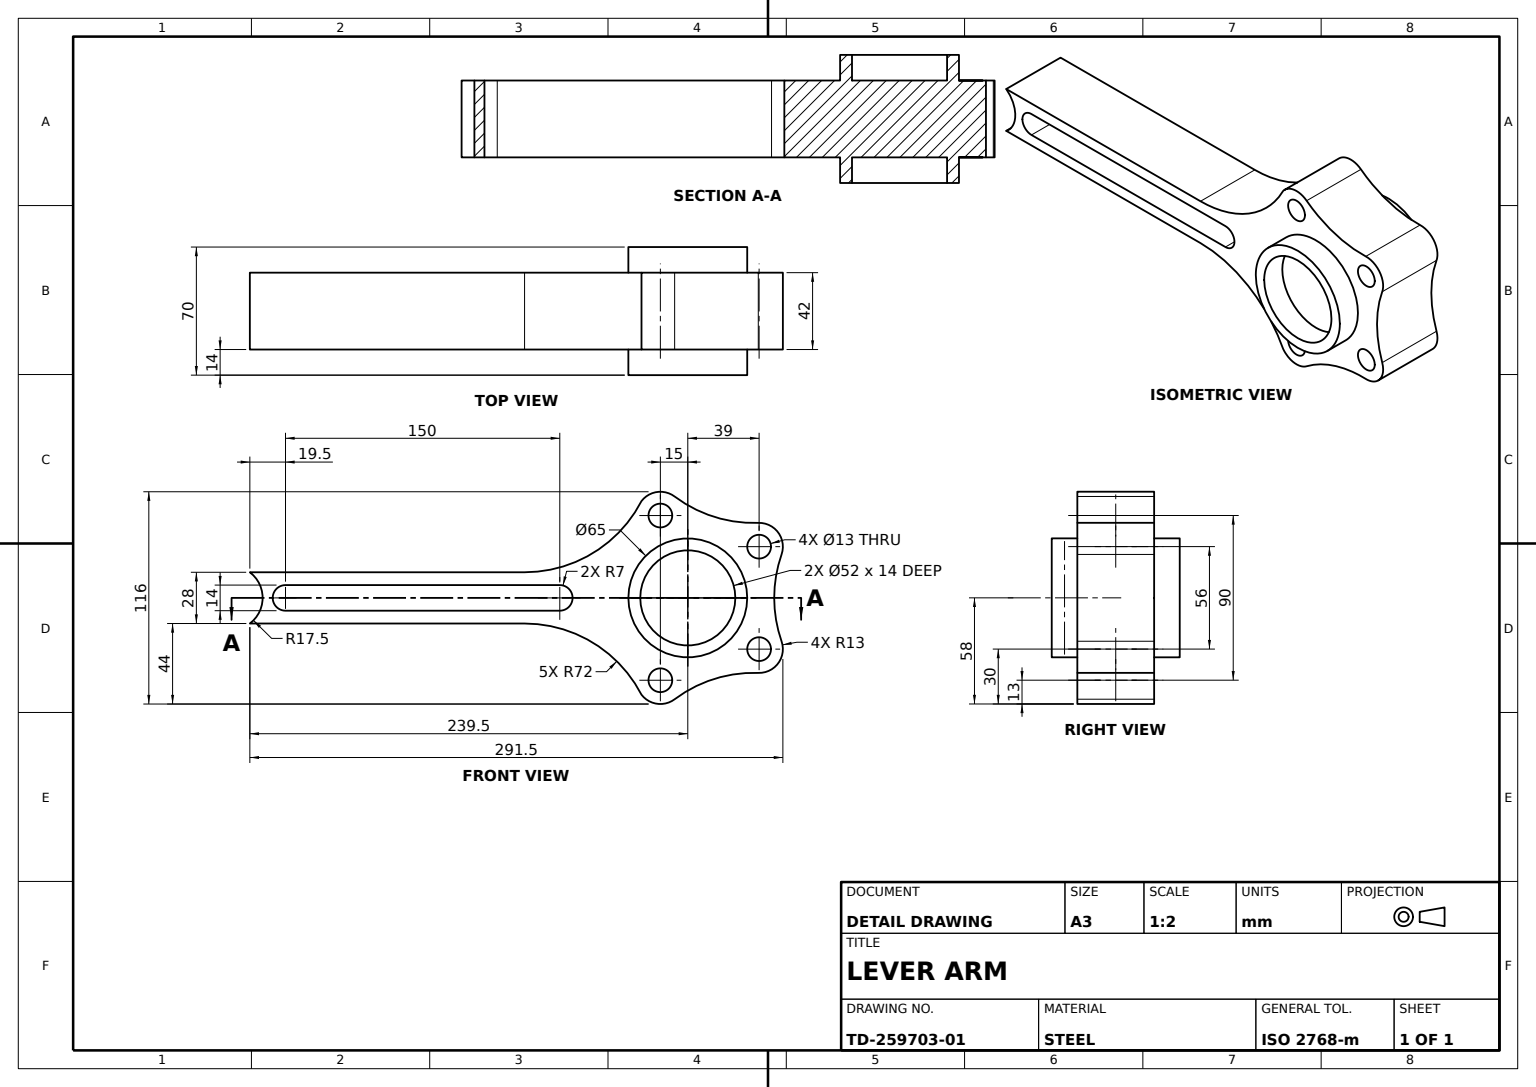
ISO-10303-21;
HEADER;
FILE_DESCRIPTION((''),'2;1');
FILE_NAME('','',(''),(''),'','','');
FILE_SCHEMA(('AUTOMOTIVE_DESIGN'));
ENDSEC;
DATA;
#1=APPLICATION_CONTEXT('');
#2=PRODUCT_CONTEXT('',#1,'mechanical');
#3=PRODUCT('','','',(#2));
#4=PRODUCT_DEFINITION_FORMATION('','',#3);
#5=PRODUCT_DEFINITION_CONTEXT('',#1,'design');
#6=PRODUCT_DEFINITION('','',#4,#5);
#7=PRODUCT_DEFINITION_SHAPE('','',#6);
#8=(LENGTH_UNIT()NAMED_UNIT(*)SI_UNIT(.MILLI.,.METRE.));
#9=(NAMED_UNIT(*)PLANE_ANGLE_UNIT()SI_UNIT($,.RADIAN.));
#10=(NAMED_UNIT(*)SI_UNIT($,.STERADIAN.)SOLID_ANGLE_UNIT());
#11=UNCERTAINTY_MEASURE_WITH_UNIT(LENGTH_MEASURE(1.E-05),#8,'distance_accuracy_value','');
#12=(GEOMETRIC_REPRESENTATION_CONTEXT(3)GLOBAL_UNCERTAINTY_ASSIGNED_CONTEXT((#11))GLOBAL_UNIT_ASSIGNED_CONTEXT((#8,#9,#10))REPRESENTATION_CONTEXT('',''));
#13=CARTESIAN_POINT('',(-70.,-7.,21.));
#14=VERTEX_POINT('',#13);
#15=CARTESIAN_POINT('',(-220.,-7.,21.));
#16=VERTEX_POINT('',#15);
#17=CARTESIAN_POINT('',(0.,-7.,21.));
#18=DIRECTION('',(-1.,0.,0.));
#19=VECTOR('',#18,1000.);
#20=LINE('',#17,#19);
#21=EDGE_CURVE('',#14,#16,#20,.T.);
#22=ORIENTED_EDGE('',*,*,#21,.F.);
#23=CARTESIAN_POINT('',(-70.,-7.,-21.));
#24=VERTEX_POINT('',#23);
#25=DIRECTION('',(0.,0.,-1.));
#26=VECTOR('',#25,1000.);
#27=LINE('',#13,#26);
#28=EDGE_CURVE('',#14,#24,#27,.T.);
#29=ORIENTED_EDGE('',*,*,#28,.T.);
#30=CARTESIAN_POINT('',(-220.,-7.,-21.));
#31=VERTEX_POINT('',#30);
#32=CARTESIAN_POINT('',(0.,-7.,-21.));
#33=LINE('',#32,#19);
#34=EDGE_CURVE('',#24,#31,#33,.T.);
#35=ORIENTED_EDGE('',*,*,#34,.T.);
#36=LINE('',#15,#26);
#37=EDGE_CURVE('',#16,#31,#36,.T.);
#38=ORIENTED_EDGE('',*,*,#37,.F.);
#39=EDGE_LOOP('',(#22,#29,#35,#38));
#40=FACE_OUTER_BOUND('',#39,.T.);
#41=DIRECTION('',(0.,-1.,0.));
#42=AXIS2_PLACEMENT_3D('',#17,#41,#25);
#43=PLANE('',#42);
#44=ADVANCED_FACE('',(#40),#43,.F.);
#45=CARTESIAN_POINT('',(26.,0.,-21.));
#46=VERTEX_POINT('',#45);
#47=CARTESIAN_POINT('',(26.,0.,-35.));
#48=VERTEX_POINT('',#47);
#49=CARTESIAN_POINT('',(26.,0.,35.));
#50=LINE('',#49,#26);
#51=EDGE_CURVE('',#46,#48,#50,.T.);
#52=ORIENTED_EDGE('',*,*,#51,.F.);
#53=CARTESIAN_POINT('',(-26.,0.,-21.));
#54=VERTEX_POINT('',#53);
#55=CARTESIAN_POINT('',(0.,0.,-21.));
#56=AXIS2_PLACEMENT_3D('',#55,#25,#18);
#57=CIRCLE('',#56,26.);
#58=EDGE_CURVE('',#54,#46,#57,.T.);
#59=ORIENTED_EDGE('',*,*,#58,.F.);
#60=CARTESIAN_POINT('',(-26.,0.,-35.));
#61=VERTEX_POINT('',#60);
#62=CARTESIAN_POINT('',(-26.,0.,35.));
#63=LINE('',#62,#26);
#64=EDGE_CURVE('',#54,#61,#63,.T.);
#65=ORIENTED_EDGE('',*,*,#64,.T.);
#66=CARTESIAN_POINT('',(0.,0.,-35.));
#67=DIRECTION('',(0.,0.,1.));
#68=DIRECTION('',(1.,0.,0.));
#69=AXIS2_PLACEMENT_3D('',#66,#67,#68);
#70=CIRCLE('',#69,26.);
#71=EDGE_CURVE('',#48,#61,#70,.T.);
#72=ORIENTED_EDGE('',*,*,#71,.F.);
#73=EDGE_LOOP('',(#52,#59,#65,#72));
#74=FACE_OUTER_BOUND('',#73,.T.);
#75=CARTESIAN_POINT('',(0.,0.,35.));
#76=AXIS2_PLACEMENT_3D('',#75,#25,#18);
#77=CYLINDRICAL_SURFACE('',#76,26.);
#78=ADVANCED_FACE('',(#74),#77,.F.);
#79=ORIENTED_EDGE('',*,*,#71,.T.);
#80=EDGE_CURVE('',#61,#48,#70,.T.);
#81=ORIENTED_EDGE('',*,*,#80,.T.);
#82=EDGE_LOOP('',(#79,#81));
#83=FACE_BOUND('',#82,.T.);
#84=CARTESIAN_POINT('',(-32.5,0.,-35.));
#85=VERTEX_POINT('',#84);
#86=CARTESIAN_POINT('',(32.5,0.,-35.));
#87=VERTEX_POINT('',#86);
#88=CIRCLE('',#69,32.5);
#89=EDGE_CURVE('',#85,#87,#88,.T.);
#90=ORIENTED_EDGE('',*,*,#89,.F.);
#91=EDGE_CURVE('',#87,#85,#88,.T.);
#92=ORIENTED_EDGE('',*,*,#91,.F.);
#93=EDGE_LOOP('',(#90,#92));
#94=FACE_OUTER_BOUND('',#93,.T.);
#95=PLANE('',#69);
#96=ADVANCED_FACE('',(#83,#94),#95,.F.);
#97=CARTESIAN_POINT('',(-89.262059,-14.,21.));
#98=VERTEX_POINT('',#97);
#99=CARTESIAN_POINT('',(-25.315909,-52.91088,21.));
#100=VERTEX_POINT('',#99);
#101=CARTESIAN_POINT('',(-89.262059,-86.,21.));
#102=AXIS2_PLACEMENT_3D('',#101,#25,#18);
#103=CIRCLE('',#102,72.);
#104=EDGE_CURVE('',#98,#100,#103,.T.);
#105=ORIENTED_EDGE('',*,*,#104,.F.);
#106=CARTESIAN_POINT('',(-89.262059,-14.,-21.));
#107=VERTEX_POINT('',#106);
#108=LINE('',#97,#26);
#109=EDGE_CURVE('',#98,#107,#108,.T.);
#110=ORIENTED_EDGE('',*,*,#109,.T.);
#111=CARTESIAN_POINT('',(-25.315909,-52.91088,-21.));
#112=VERTEX_POINT('',#111);
#113=CARTESIAN_POINT('',(-89.262059,-86.,-21.));
#114=AXIS2_PLACEMENT_3D('',#113,#25,#18);
#115=CIRCLE('',#114,72.);
#116=EDGE_CURVE('',#107,#112,#115,.T.);
#117=ORIENTED_EDGE('',*,*,#116,.T.);
#118=LINE('',#99,#26);
#119=EDGE_CURVE('',#100,#112,#118,.T.);
#120=ORIENTED_EDGE('',*,*,#119,.F.);
#121=EDGE_LOOP('',(#105,#110,#117,#120));
#122=FACE_OUTER_BOUND('',#121,.T.);
#123=CYLINDRICAL_SURFACE('',#102,72.);
#124=ADVANCED_FACE('',(#122),#123,.F.);
#125=CARTESIAN_POINT('',(45.5,-28.,21.));
#126=VERTEX_POINT('',#125);
#127=CARTESIAN_POINT('',(45.5,-28.,-21.));
#128=VERTEX_POINT('',#127);
#129=LINE('',#125,#26);
#130=EDGE_CURVE('',#126,#128,#129,.T.);
#131=ORIENTED_EDGE('',*,*,#130,.T.);
#132=CARTESIAN_POINT('',(32.5,-28.,-21.));
#133=VERTEX_POINT('',#132);
#134=CARTESIAN_POINT('',(39.,-28.,-21.));
#135=AXIS2_PLACEMENT_3D('',#134,#25,#18);
#136=CIRCLE('',#135,6.5);
#137=EDGE_CURVE('',#128,#133,#136,.T.);
#138=ORIENTED_EDGE('',*,*,#137,.T.);
#139=CARTESIAN_POINT('',(32.5,-28.,21.));
#140=VERTEX_POINT('',#139);
#141=LINE('',#139,#26);
#142=EDGE_CURVE('',#140,#133,#141,.T.);
#143=ORIENTED_EDGE('',*,*,#142,.F.);
#144=CARTESIAN_POINT('',(39.,-28.,21.));
#145=AXIS2_PLACEMENT_3D('',#144,#25,#18);
#146=CIRCLE('',#145,6.5);
#147=EDGE_CURVE('',#126,#140,#146,.T.);
#148=ORIENTED_EDGE('',*,*,#147,.F.);
#149=EDGE_LOOP('',(#131,#138,#143,#148));
#150=FACE_OUTER_BOUND('',#149,.T.);
#151=CYLINDRICAL_SURFACE('',#145,6.5);
#152=ADVANCED_FACE('',(#150),#151,.F.);
#153=CARTESIAN_POINT('',(-7.189691,-55.392261,21.));
#154=VERTEX_POINT('',#153);
#155=CARTESIAN_POINT('',(-7.189691,-55.392261,-21.));
#156=VERTEX_POINT('',#155);
#157=LINE('',#153,#26);
#158=EDGE_CURVE('',#154,#156,#157,.T.);
#159=ORIENTED_EDGE('',*,*,#158,.T.);
#160=CARTESIAN_POINT('',(38.551485,-40.992261,-21.));
#161=VERTEX_POINT('',#160);
#162=CARTESIAN_POINT('',(36.067402,-112.949396,-21.));
#163=AXIS2_PLACEMENT_3D('',#162,#25,#18);
#164=CIRCLE('',#163,72.);
#165=EDGE_CURVE('',#156,#161,#164,.T.);
#166=ORIENTED_EDGE('',*,*,#165,.T.);
#167=CARTESIAN_POINT('',(38.551485,-40.992261,21.));
#168=VERTEX_POINT('',#167);
#169=LINE('',#167,#26);
#170=EDGE_CURVE('',#168,#161,#169,.T.);
#171=ORIENTED_EDGE('',*,*,#170,.F.);
#172=CARTESIAN_POINT('',(36.067402,-112.949396,21.));
#173=AXIS2_PLACEMENT_3D('',#172,#25,#18);
#174=CIRCLE('',#173,72.);
#175=EDGE_CURVE('',#154,#168,#174,.T.);
#176=ORIENTED_EDGE('',*,*,#175,.F.);
#177=EDGE_LOOP('',(#159,#166,#171,#176));
#178=FACE_OUTER_BOUND('',#177,.T.);
#179=CYLINDRICAL_SURFACE('',#173,72.);
#180=ADVANCED_FACE('',(#178),#179,.F.);
#181=EDGE_CURVE('',#46,#54,#57,.T.);
#182=ORIENTED_EDGE('',*,*,#181,.T.);
#183=ORIENTED_EDGE('',*,*,#58,.T.);
#184=EDGE_LOOP('',(#182,#183));
#185=FACE_OUTER_BOUND('',#184,.T.);
#186=PLANE('',#56);
#187=ADVANCED_FACE('',(#185),#186,.T.);
#188=CARTESIAN_POINT('',(-25.315909,52.91088,21.));
#189=VERTEX_POINT('',#188);
#190=CARTESIAN_POINT('',(-7.189691,55.392261,21.));
#191=VERTEX_POINT('',#190);
#192=CARTESIAN_POINT('',(-15.,45.,21.));
#193=AXIS2_PLACEMENT_3D('',#192,#25,#18);
#194=CIRCLE('',#193,13.);
#195=EDGE_CURVE('',#189,#191,#194,.T.);
#196=ORIENTED_EDGE('',*,*,#195,.T.);
#197=CARTESIAN_POINT('',(-7.189691,55.392261,-21.));
#198=VERTEX_POINT('',#197);
#199=LINE('',#190,#26);
#200=EDGE_CURVE('',#191,#198,#199,.T.);
#201=ORIENTED_EDGE('',*,*,#200,.T.);
#202=CARTESIAN_POINT('',(-25.315909,52.91088,-21.));
#203=VERTEX_POINT('',#202);
#204=CARTESIAN_POINT('',(-15.,45.,-21.));
#205=AXIS2_PLACEMENT_3D('',#204,#25,#18);
#206=CIRCLE('',#205,13.);
#207=EDGE_CURVE('',#203,#198,#206,.T.);
#208=ORIENTED_EDGE('',*,*,#207,.F.);
#209=LINE('',#188,#26);
#210=EDGE_CURVE('',#189,#203,#209,.T.);
#211=ORIENTED_EDGE('',*,*,#210,.F.);
#212=EDGE_LOOP('',(#196,#201,#208,#211));
#213=FACE_OUTER_BOUND('',#212,.T.);
#214=CYLINDRICAL_SURFACE('',#193,13.);
#215=ADVANCED_FACE('',(#213),#214,.T.);
#216=CARTESIAN_POINT('',(-21.5,-45.,-21.));
#217=VERTEX_POINT('',#216);
#218=CARTESIAN_POINT('',(-8.5,-45.,-21.));
#219=VERTEX_POINT('',#218);
#220=CARTESIAN_POINT('',(-15.,-45.,-21.));
#221=AXIS2_PLACEMENT_3D('',#220,#25,#18);
#222=CIRCLE('',#221,6.5);
#223=EDGE_CURVE('',#217,#219,#222,.T.);
#224=ORIENTED_EDGE('',*,*,#223,.T.);
#225=CARTESIAN_POINT('',(-8.5,-45.,21.));
#226=VERTEX_POINT('',#225);
#227=LINE('',#225,#26);
#228=EDGE_CURVE('',#226,#219,#227,.T.);
#229=ORIENTED_EDGE('',*,*,#228,.F.);
#230=CARTESIAN_POINT('',(-21.5,-45.,21.));
#231=VERTEX_POINT('',#230);
#232=CARTESIAN_POINT('',(-15.,-45.,21.));
#233=AXIS2_PLACEMENT_3D('',#232,#25,#18);
#234=CIRCLE('',#233,6.5);
#235=EDGE_CURVE('',#231,#226,#234,.T.);
#236=ORIENTED_EDGE('',*,*,#235,.F.);
#237=LINE('',#230,#26);
#238=EDGE_CURVE('',#231,#217,#237,.T.);
#239=ORIENTED_EDGE('',*,*,#238,.T.);
#240=EDGE_LOOP('',(#224,#229,#236,#239));
#241=FACE_OUTER_BOUND('',#240,.T.);
#242=CYLINDRICAL_SURFACE('',#233,6.5);
#243=ADVANCED_FACE('',(#241),#242,.F.);
#244=CARTESIAN_POINT('',(32.5,28.,21.));
#245=VERTEX_POINT('',#244);
#246=CARTESIAN_POINT('',(45.5,28.,21.));
#247=VERTEX_POINT('',#246);
#248=CARTESIAN_POINT('',(39.,28.,21.));
#249=AXIS2_PLACEMENT_3D('',#248,#25,#18);
#250=CIRCLE('',#249,6.5);
#251=EDGE_CURVE('',#245,#247,#250,.T.);
#252=ORIENTED_EDGE('',*,*,#251,.F.);
#253=CARTESIAN_POINT('',(32.5,28.,-21.));
#254=VERTEX_POINT('',#253);
#255=LINE('',#244,#26);
#256=EDGE_CURVE('',#245,#254,#255,.T.);
#257=ORIENTED_EDGE('',*,*,#256,.T.);
#258=CARTESIAN_POINT('',(45.5,28.,-21.));
#259=VERTEX_POINT('',#258);
#260=CARTESIAN_POINT('',(39.,28.,-21.));
#261=AXIS2_PLACEMENT_3D('',#260,#25,#18);
#262=CIRCLE('',#261,6.5);
#263=EDGE_CURVE('',#254,#259,#262,.T.);
#264=ORIENTED_EDGE('',*,*,#263,.T.);
#265=LINE('',#246,#26);
#266=EDGE_CURVE('',#247,#259,#265,.T.);
#267=ORIENTED_EDGE('',*,*,#266,.F.);
#268=EDGE_LOOP('',(#252,#257,#264,#267));
#269=FACE_OUTER_BOUND('',#268,.T.);
#270=CYLINDRICAL_SURFACE('',#249,6.5);
#271=ADVANCED_FACE('',(#269),#270,.F.);
#272=ORIENTED_EDGE('',*,*,#238,.F.);
#273=EDGE_CURVE('',#226,#231,#234,.T.);
#274=ORIENTED_EDGE('',*,*,#273,.F.);
#275=ORIENTED_EDGE('',*,*,#228,.T.);
#276=EDGE_CURVE('',#219,#217,#222,.T.);
#277=ORIENTED_EDGE('',*,*,#276,.T.);
#278=EDGE_LOOP('',(#272,#274,#275,#277));
#279=FACE_OUTER_BOUND('',#278,.T.);
#280=ADVANCED_FACE('',(#279),#242,.F.);
#281=ORIENTED_EDGE('',*,*,#37,.T.);
#282=CARTESIAN_POINT('',(-227.,0.,-21.));
#283=VERTEX_POINT('',#282);
#284=CARTESIAN_POINT('',(-220.,0.,-21.));
#285=AXIS2_PLACEMENT_3D('',#284,#25,#18);
#286=CIRCLE('',#285,7.);
#287=EDGE_CURVE('',#31,#283,#286,.T.);
#288=ORIENTED_EDGE('',*,*,#287,.T.);
#289=CARTESIAN_POINT('',(-227.,0.,21.));
#290=VERTEX_POINT('',#289);
#291=LINE('',#289,#26);
#292=EDGE_CURVE('',#290,#283,#291,.T.);
#293=ORIENTED_EDGE('',*,*,#292,.F.);
#294=CARTESIAN_POINT('',(-220.,0.,21.));
#295=AXIS2_PLACEMENT_3D('',#294,#25,#18);
#296=CIRCLE('',#295,7.);
#297=EDGE_CURVE('',#16,#290,#296,.T.);
#298=ORIENTED_EDGE('',*,*,#297,.F.);
#299=EDGE_LOOP('',(#281,#288,#293,#298));
#300=FACE_OUTER_BOUND('',#299,.T.);
#301=CYLINDRICAL_SURFACE('',#295,7.);
#302=ADVANCED_FACE('',(#300),#301,.F.);
#303=CARTESIAN_POINT('',(-89.262059,14.,-21.));
#304=VERTEX_POINT('',#303);
#305=CARTESIAN_POINT('',(-89.262059,86.,-21.));
#306=AXIS2_PLACEMENT_3D('',#305,#25,#18);
#307=CIRCLE('',#306,72.);
#308=EDGE_CURVE('',#203,#304,#307,.T.);
#309=ORIENTED_EDGE('',*,*,#308,.T.);
#310=CARTESIAN_POINT('',(-89.262059,14.,21.));
#311=VERTEX_POINT('',#310);
#312=LINE('',#310,#26);
#313=EDGE_CURVE('',#311,#304,#312,.T.);
#314=ORIENTED_EDGE('',*,*,#313,.F.);
#315=CARTESIAN_POINT('',(-89.262059,86.,21.));
#316=AXIS2_PLACEMENT_3D('',#315,#25,#18);
#317=CIRCLE('',#316,72.);
#318=EDGE_CURVE('',#189,#311,#317,.T.);
#319=ORIENTED_EDGE('',*,*,#318,.F.);
#320=ORIENTED_EDGE('',*,*,#210,.T.);
#321=EDGE_LOOP('',(#309,#314,#319,#320));
#322=FACE_OUTER_BOUND('',#321,.T.);
#323=CYLINDRICAL_SURFACE('',#316,72.);
#324=ADVANCED_FACE('',(#322),#323,.F.);
#325=VERTEX_POINT('',#62);
#326=VERTEX_POINT('',#49);
#327=AXIS2_PLACEMENT_3D('',#75,#67,#68);
#328=CIRCLE('',#327,26.);
#329=EDGE_CURVE('',#325,#326,#328,.T.);
#330=ORIENTED_EDGE('',*,*,#329,.T.);
#331=CARTESIAN_POINT('',(26.,0.,21.));
#332=VERTEX_POINT('',#331);
#333=EDGE_CURVE('',#326,#332,#50,.T.);
#334=ORIENTED_EDGE('',*,*,#333,.T.);
#335=CARTESIAN_POINT('',(-26.,0.,21.));
#336=VERTEX_POINT('',#335);
#337=CARTESIAN_POINT('',(0.,0.,21.));
#338=AXIS2_PLACEMENT_3D('',#337,#25,#18);
#339=CIRCLE('',#338,26.);
#340=EDGE_CURVE('',#332,#336,#339,.T.);
#341=ORIENTED_EDGE('',*,*,#340,.T.);
#342=EDGE_CURVE('',#325,#336,#63,.T.);
#343=ORIENTED_EDGE('',*,*,#342,.F.);
#344=EDGE_LOOP('',(#330,#334,#341,#343));
#345=FACE_OUTER_BOUND('',#344,.T.);
#346=ADVANCED_FACE('',(#345),#77,.F.);
#347=ORIENTED_EDGE('',*,*,#130,.F.);
#348=EDGE_CURVE('',#140,#126,#146,.T.);
#349=ORIENTED_EDGE('',*,*,#348,.F.);
#350=ORIENTED_EDGE('',*,*,#142,.T.);
#351=EDGE_CURVE('',#133,#128,#136,.T.);
#352=ORIENTED_EDGE('',*,*,#351,.T.);
#353=EDGE_LOOP('',(#347,#349,#350,#352));
#354=FACE_OUTER_BOUND('',#353,.T.);
#355=ADVANCED_FACE('',(#354),#151,.F.);
#356=CARTESIAN_POINT('',(-8.5,45.,-21.));
#357=VERTEX_POINT('',#356);
#358=CARTESIAN_POINT('',(-21.5,45.,-21.));
#359=VERTEX_POINT('',#358);
#360=CIRCLE('',#205,6.5);
#361=EDGE_CURVE('',#357,#359,#360,.T.);
#362=ORIENTED_EDGE('',*,*,#361,.F.);
#363=EDGE_CURVE('',#359,#357,#360,.T.);
#364=ORIENTED_EDGE('',*,*,#363,.F.);
#365=EDGE_LOOP('',(#362,#364));
#366=FACE_BOUND('',#365,.T.);
#367=ORIENTED_EDGE('',*,*,#137,.F.);
#368=ORIENTED_EDGE('',*,*,#351,.F.);
#369=EDGE_LOOP('',(#367,#368));
#370=FACE_BOUND('',#369,.T.);
#371=CIRCLE('',#221,13.);
#372=EDGE_CURVE('',#156,#112,#371,.T.);
#373=ORIENTED_EDGE('',*,*,#372,.T.);
#374=ORIENTED_EDGE('',*,*,#116,.F.);
#375=CARTESIAN_POINT('',(-239.5,-14.,-21.));
#376=VERTEX_POINT('',#375);
#377=CARTESIAN_POINT('',(0.,-14.,-21.));
#378=VECTOR('',#68,1000.);
#379=LINE('',#377,#378);
#380=EDGE_CURVE('',#376,#107,#379,.T.);
#381=ORIENTED_EDGE('',*,*,#380,.F.);
#382=CARTESIAN_POINT('',(-239.5,14.,-21.));
#383=VERTEX_POINT('',#382);
#384=CARTESIAN_POINT('',(-250.,0.,-21.));
#385=AXIS2_PLACEMENT_3D('',#384,#25,#18);
#386=CIRCLE('',#385,17.5);
#387=EDGE_CURVE('',#383,#376,#386,.T.);
#388=ORIENTED_EDGE('',*,*,#387,.F.);
#389=CARTESIAN_POINT('',(0.,14.,-21.));
#390=LINE('',#389,#19);
#391=EDGE_CURVE('',#304,#383,#390,.T.);
#392=ORIENTED_EDGE('',*,*,#391,.F.);
#393=ORIENTED_EDGE('',*,*,#308,.F.);
#394=ORIENTED_EDGE('',*,*,#207,.T.);
#395=CARTESIAN_POINT('',(38.551485,40.992261,-21.));
#396=VERTEX_POINT('',#395);
#397=CARTESIAN_POINT('',(36.067402,112.949396,-21.));
#398=AXIS2_PLACEMENT_3D('',#397,#25,#18);
#399=CIRCLE('',#398,72.);
#400=EDGE_CURVE('',#396,#198,#399,.T.);
#401=ORIENTED_EDGE('',*,*,#400,.F.);
#402=CARTESIAN_POINT('',(51.274423,23.717647,-21.));
#403=VERTEX_POINT('',#402);
#404=CIRCLE('',#261,13.);
#405=EDGE_CURVE('',#396,#403,#404,.T.);
#406=ORIENTED_EDGE('',*,*,#405,.T.);
#407=CARTESIAN_POINT('',(47.255841,0.,-21.));
#408=VERTEX_POINT('',#407);
#409=CARTESIAN_POINT('',(119.255841,0.,-21.));
#410=AXIS2_PLACEMENT_3D('',#409,#25,#18);
#411=CIRCLE('',#410,72.);
#412=EDGE_CURVE('',#408,#403,#411,.T.);
#413=ORIENTED_EDGE('',*,*,#412,.F.);
#414=CARTESIAN_POINT('',(51.274423,-23.717647,-21.));
#415=VERTEX_POINT('',#414);
#416=EDGE_CURVE('',#415,#408,#411,.T.);
#417=ORIENTED_EDGE('',*,*,#416,.F.);
#418=CIRCLE('',#135,13.);
#419=EDGE_CURVE('',#415,#161,#418,.T.);
#420=ORIENTED_EDGE('',*,*,#419,.T.);
#421=ORIENTED_EDGE('',*,*,#165,.F.);
#422=EDGE_LOOP('',(#373,#374,#381,#388,#392,#393,#394,#401,#406,#413,#417,#420,#421));
#423=FACE_OUTER_BOUND('',#422,.T.);
#424=EDGE_CURVE('',#259,#254,#262,.T.);
#425=ORIENTED_EDGE('',*,*,#424,.F.);
#426=ORIENTED_EDGE('',*,*,#263,.F.);
#427=EDGE_LOOP('',(#425,#426));
#428=FACE_BOUND('',#427,.T.);
#429=CARTESIAN_POINT('',(-70.,7.,-21.));
#430=VERTEX_POINT('',#429);
#431=CARTESIAN_POINT('',(-220.,7.,-21.));
#432=VERTEX_POINT('',#431);
#433=CARTESIAN_POINT('',(0.,7.,-21.));
#434=LINE('',#433,#19);
#435=EDGE_CURVE('',#430,#432,#434,.T.);
#436=ORIENTED_EDGE('',*,*,#435,.T.);
#437=EDGE_CURVE('',#283,#432,#286,.T.);
#438=ORIENTED_EDGE('',*,*,#437,.F.);
#439=ORIENTED_EDGE('',*,*,#287,.F.);
#440=ORIENTED_EDGE('',*,*,#34,.F.);
#441=CARTESIAN_POINT('',(-70.,0.,-21.));
#442=AXIS2_PLACEMENT_3D('',#441,#25,#18);
#443=CIRCLE('',#442,7.);
#444=EDGE_CURVE('',#430,#24,#443,.T.);
#445=ORIENTED_EDGE('',*,*,#444,.F.);
#446=EDGE_LOOP('',(#436,#438,#439,#440,#445));
#447=FACE_BOUND('',#446,.T.);
#448=ORIENTED_EDGE('',*,*,#223,.F.);
#449=ORIENTED_EDGE('',*,*,#276,.F.);
#450=EDGE_LOOP('',(#448,#449));
#451=FACE_BOUND('',#450,.T.);
#452=CARTESIAN_POINT('',(-32.5,0.,-21.));
#453=VERTEX_POINT('',#452);
#454=CARTESIAN_POINT('',(32.5,0.,-21.));
#455=VERTEX_POINT('',#454);
#456=CIRCLE('',#56,32.5);
#457=EDGE_CURVE('',#453,#455,#456,.T.);
#458=ORIENTED_EDGE('',*,*,#457,.F.);
#459=EDGE_CURVE('',#455,#453,#456,.T.);
#460=ORIENTED_EDGE('',*,*,#459,.F.);
#461=EDGE_LOOP('',(#458,#460));
#462=FACE_BOUND('',#461,.T.);
#463=ADVANCED_FACE('',(#366,#370,#423,#428,#447,#451,#462),#186,.T.);
#464=CARTESIAN_POINT('',(51.274423,-23.717647,21.));
#465=VERTEX_POINT('',#464);
#466=CIRCLE('',#145,13.);
#467=EDGE_CURVE('',#465,#168,#466,.T.);
#468=ORIENTED_EDGE('',*,*,#467,.T.);
#469=ORIENTED_EDGE('',*,*,#170,.T.);
#470=ORIENTED_EDGE('',*,*,#419,.F.);
#471=LINE('',#464,#26);
#472=EDGE_CURVE('',#465,#415,#471,.T.);
#473=ORIENTED_EDGE('',*,*,#472,.F.);
#474=EDGE_LOOP('',(#468,#469,#470,#473));
#475=FACE_OUTER_BOUND('',#474,.T.);
#476=CYLINDRICAL_SURFACE('',#145,13.);
#477=ADVANCED_FACE('',(#475),#476,.T.);
#478=CARTESIAN_POINT('',(-220.,7.,21.));
#479=VERTEX_POINT('',#478);
#480=LINE('',#478,#26);
#481=EDGE_CURVE('',#479,#432,#480,.T.);
#482=ORIENTED_EDGE('',*,*,#481,.F.);
#483=EDGE_CURVE('',#290,#479,#296,.T.);
#484=ORIENTED_EDGE('',*,*,#483,.F.);
#485=ORIENTED_EDGE('',*,*,#292,.T.);
#486=ORIENTED_EDGE('',*,*,#437,.T.);
#487=EDGE_LOOP('',(#482,#484,#485,#486));
#488=FACE_OUTER_BOUND('',#487,.T.);
#489=ADVANCED_FACE('',(#488),#301,.F.);
#490=CARTESIAN_POINT('',(-8.5,45.,21.));
#491=VERTEX_POINT('',#490);
#492=LINE('',#490,#26);
#493=EDGE_CURVE('',#491,#357,#492,.T.);
#494=ORIENTED_EDGE('',*,*,#493,.T.);
#495=ORIENTED_EDGE('',*,*,#361,.T.);
#496=CARTESIAN_POINT('',(-21.5,45.,21.));
#497=VERTEX_POINT('',#496);
#498=LINE('',#496,#26);
#499=EDGE_CURVE('',#497,#359,#498,.T.);
#500=ORIENTED_EDGE('',*,*,#499,.F.);
#501=CIRCLE('',#193,6.5);
#502=EDGE_CURVE('',#491,#497,#501,.T.);
#503=ORIENTED_EDGE('',*,*,#502,.F.);
#504=EDGE_LOOP('',(#494,#495,#500,#503));
#505=FACE_OUTER_BOUND('',#504,.T.);
#506=CYLINDRICAL_SURFACE('',#193,6.5);
#507=ADVANCED_FACE('',(#505),#506,.F.);
#508=CARTESIAN_POINT('',(-32.5,0.,21.));
#509=VERTEX_POINT('',#508);
#510=CARTESIAN_POINT('',(32.5,0.,21.));
#511=VERTEX_POINT('',#510);
#512=CIRCLE('',#338,32.5);
#513=EDGE_CURVE('',#509,#511,#512,.T.);
#514=ORIENTED_EDGE('',*,*,#513,.T.);
#515=EDGE_CURVE('',#511,#509,#512,.T.);
#516=ORIENTED_EDGE('',*,*,#515,.T.);
#517=EDGE_LOOP('',(#514,#516));
#518=FACE_BOUND('',#517,.T.);
#519=ORIENTED_EDGE('',*,*,#104,.T.);
#520=CIRCLE('',#233,13.);
#521=EDGE_CURVE('',#154,#100,#520,.T.);
#522=ORIENTED_EDGE('',*,*,#521,.F.);
#523=ORIENTED_EDGE('',*,*,#175,.T.);
#524=ORIENTED_EDGE('',*,*,#467,.F.);
#525=CARTESIAN_POINT('',(47.255841,0.,21.));
#526=VERTEX_POINT('',#525);
#527=CARTESIAN_POINT('',(119.255841,0.,21.));
#528=AXIS2_PLACEMENT_3D('',#527,#25,#18);
#529=CIRCLE('',#528,72.);
#530=EDGE_CURVE('',#465,#526,#529,.T.);
#531=ORIENTED_EDGE('',*,*,#530,.T.);
#532=CARTESIAN_POINT('',(51.274423,23.717647,21.));
#533=VERTEX_POINT('',#532);
#534=EDGE_CURVE('',#526,#533,#529,.T.);
#535=ORIENTED_EDGE('',*,*,#534,.T.);
#536=CARTESIAN_POINT('',(38.551485,40.992261,21.));
#537=VERTEX_POINT('',#536);
#538=CIRCLE('',#249,13.);
#539=EDGE_CURVE('',#537,#533,#538,.T.);
#540=ORIENTED_EDGE('',*,*,#539,.F.);
#541=CARTESIAN_POINT('',(36.067402,112.949396,21.));
#542=AXIS2_PLACEMENT_3D('',#541,#25,#18);
#543=CIRCLE('',#542,72.);
#544=EDGE_CURVE('',#537,#191,#543,.T.);
#545=ORIENTED_EDGE('',*,*,#544,.T.);
#546=ORIENTED_EDGE('',*,*,#195,.F.);
#547=ORIENTED_EDGE('',*,*,#318,.T.);
#548=CARTESIAN_POINT('',(-239.5,14.,21.));
#549=VERTEX_POINT('',#548);
#550=CARTESIAN_POINT('',(0.,14.,21.));
#551=LINE('',#550,#19);
#552=EDGE_CURVE('',#311,#549,#551,.T.);
#553=ORIENTED_EDGE('',*,*,#552,.T.);
#554=CARTESIAN_POINT('',(-239.5,-14.,21.));
#555=VERTEX_POINT('',#554);
#556=CARTESIAN_POINT('',(-250.,0.,21.));
#557=AXIS2_PLACEMENT_3D('',#556,#25,#18);
#558=CIRCLE('',#557,17.5);
#559=EDGE_CURVE('',#549,#555,#558,.T.);
#560=ORIENTED_EDGE('',*,*,#559,.T.);
#561=CARTESIAN_POINT('',(0.,-14.,21.));
#562=LINE('',#561,#378);
#563=EDGE_CURVE('',#555,#98,#562,.T.);
#564=ORIENTED_EDGE('',*,*,#563,.T.);
#565=EDGE_LOOP('',(#519,#522,#523,#524,#531,#535,#540,#545,#546,#547,#553,#560,#564));
#566=FACE_OUTER_BOUND('',#565,.T.);
#567=ORIENTED_EDGE('',*,*,#502,.T.);
#568=EDGE_CURVE('',#497,#491,#501,.T.);
#569=ORIENTED_EDGE('',*,*,#568,.T.);
#570=EDGE_LOOP('',(#567,#569));
#571=FACE_BOUND('',#570,.T.);
#572=ORIENTED_EDGE('',*,*,#21,.T.);
#573=ORIENTED_EDGE('',*,*,#297,.T.);
#574=ORIENTED_EDGE('',*,*,#483,.T.);
#575=CARTESIAN_POINT('',(-70.,7.,21.));
#576=VERTEX_POINT('',#575);
#577=CARTESIAN_POINT('',(0.,7.,21.));
#578=LINE('',#577,#19);
#579=EDGE_CURVE('',#576,#479,#578,.T.);
#580=ORIENTED_EDGE('',*,*,#579,.F.);
#581=CARTESIAN_POINT('',(-70.,0.,21.));
#582=AXIS2_PLACEMENT_3D('',#581,#25,#18);
#583=CIRCLE('',#582,7.);
#584=EDGE_CURVE('',#576,#14,#583,.T.);
#585=ORIENTED_EDGE('',*,*,#584,.T.);
#586=EDGE_LOOP('',(#572,#573,#574,#580,#585));
#587=FACE_BOUND('',#586,.T.);
#588=ORIENTED_EDGE('',*,*,#251,.T.);
#589=EDGE_CURVE('',#247,#245,#250,.T.);
#590=ORIENTED_EDGE('',*,*,#589,.T.);
#591=EDGE_LOOP('',(#588,#590));
#592=FACE_BOUND('',#591,.T.);
#593=ORIENTED_EDGE('',*,*,#273,.T.);
#594=ORIENTED_EDGE('',*,*,#235,.T.);
#595=EDGE_LOOP('',(#593,#594));
#596=FACE_BOUND('',#595,.T.);
#597=ORIENTED_EDGE('',*,*,#348,.T.);
#598=ORIENTED_EDGE('',*,*,#147,.T.);
#599=EDGE_LOOP('',(#597,#598));
#600=FACE_BOUND('',#599,.T.);
#601=PLANE('',#338);
#602=ADVANCED_FACE('',(#518,#566,#571,#587,#592,#596,#600),#601,.F.);
#603=CARTESIAN_POINT('',(32.5,0.,35.));
#604=VERTEX_POINT('',#603);
#605=CARTESIAN_POINT('',(-32.5,0.,35.));
#606=VERTEX_POINT('',#605);
#607=CIRCLE('',#327,32.5);
#608=EDGE_CURVE('',#604,#606,#607,.T.);
#609=ORIENTED_EDGE('',*,*,#608,.F.);
#610=LINE('',#603,#26);
#611=EDGE_CURVE('',#604,#511,#610,.T.);
#612=ORIENTED_EDGE('',*,*,#611,.T.);
#613=ORIENTED_EDGE('',*,*,#513,.F.);
#614=LINE('',#605,#26);
#615=EDGE_CURVE('',#606,#509,#614,.T.);
#616=ORIENTED_EDGE('',*,*,#615,.F.);
#617=EDGE_LOOP('',(#609,#612,#613,#616));
#618=FACE_OUTER_BOUND('',#617,.T.);
#619=CYLINDRICAL_SURFACE('',#76,32.5);
#620=ADVANCED_FACE('',(#618),#619,.T.);
#621=ORIENTED_EDGE('',*,*,#579,.T.);
#622=ORIENTED_EDGE('',*,*,#481,.T.);
#623=ORIENTED_EDGE('',*,*,#435,.F.);
#624=LINE('',#575,#26);
#625=EDGE_CURVE('',#576,#430,#624,.T.);
#626=ORIENTED_EDGE('',*,*,#625,.F.);
#627=EDGE_LOOP('',(#621,#622,#623,#626));
#628=FACE_OUTER_BOUND('',#627,.T.);
#629=AXIS2_PLACEMENT_3D('',#577,#41,#25);
#630=PLANE('',#629);
#631=ADVANCED_FACE('',(#628),#630,.T.);
#632=ORIENTED_EDGE('',*,*,#457,.T.);
#633=EDGE_CURVE('',#455,#87,#610,.T.);
#634=ORIENTED_EDGE('',*,*,#633,.T.);
#635=ORIENTED_EDGE('',*,*,#91,.T.);
#636=EDGE_CURVE('',#453,#85,#614,.T.);
#637=ORIENTED_EDGE('',*,*,#636,.F.);
#638=EDGE_LOOP('',(#632,#634,#635,#637));
#639=FACE_OUTER_BOUND('',#638,.T.);
#640=ADVANCED_FACE('',(#639),#619,.T.);
#641=ORIENTED_EDGE('',*,*,#340,.F.);
#642=EDGE_CURVE('',#336,#332,#339,.T.);
#643=ORIENTED_EDGE('',*,*,#642,.F.);
#644=EDGE_LOOP('',(#641,#643));
#645=FACE_OUTER_BOUND('',#644,.T.);
#646=ADVANCED_FACE('',(#645),#601,.F.);
#647=LINE('',#554,#26);
#648=EDGE_CURVE('',#555,#376,#647,.T.);
#649=ORIENTED_EDGE('',*,*,#648,.F.);
#650=ORIENTED_EDGE('',*,*,#559,.F.);
#651=LINE('',#548,#26);
#652=EDGE_CURVE('',#549,#383,#651,.T.);
#653=ORIENTED_EDGE('',*,*,#652,.T.);
#654=ORIENTED_EDGE('',*,*,#387,.T.);
#655=EDGE_LOOP('',(#649,#650,#653,#654));
#656=FACE_OUTER_BOUND('',#655,.T.);
#657=CYLINDRICAL_SURFACE('',#557,17.5);
#658=ADVANCED_FACE('',(#656),#657,.F.);
#659=ORIENTED_EDGE('',*,*,#391,.T.);
#660=ORIENTED_EDGE('',*,*,#652,.F.);
#661=ORIENTED_EDGE('',*,*,#552,.F.);
#662=ORIENTED_EDGE('',*,*,#313,.T.);
#663=EDGE_LOOP('',(#659,#660,#661,#662));
#664=FACE_OUTER_BOUND('',#663,.T.);
#665=AXIS2_PLACEMENT_3D('',#550,#41,#68);
#666=PLANE('',#665);
#667=ADVANCED_FACE('',(#664),#666,.F.);
#668=ORIENTED_EDGE('',*,*,#444,.T.);
#669=ORIENTED_EDGE('',*,*,#28,.F.);
#670=ORIENTED_EDGE('',*,*,#584,.F.);
#671=ORIENTED_EDGE('',*,*,#625,.T.);
#672=EDGE_LOOP('',(#668,#669,#670,#671));
#673=FACE_OUTER_BOUND('',#672,.T.);
#674=CYLINDRICAL_SURFACE('',#582,7.);
#675=ADVANCED_FACE('',(#673),#674,.F.);
#676=ORIENTED_EDGE('',*,*,#615,.T.);
#677=ORIENTED_EDGE('',*,*,#515,.F.);
#678=ORIENTED_EDGE('',*,*,#611,.F.);
#679=EDGE_CURVE('',#606,#604,#607,.T.);
#680=ORIENTED_EDGE('',*,*,#679,.F.);
#681=EDGE_LOOP('',(#676,#677,#678,#680));
#682=FACE_OUTER_BOUND('',#681,.T.);
#683=ADVANCED_FACE('',(#682),#619,.T.);
#684=ORIENTED_EDGE('',*,*,#539,.T.);
#685=LINE('',#532,#26);
#686=EDGE_CURVE('',#533,#403,#685,.T.);
#687=ORIENTED_EDGE('',*,*,#686,.T.);
#688=ORIENTED_EDGE('',*,*,#405,.F.);
#689=LINE('',#536,#26);
#690=EDGE_CURVE('',#537,#396,#689,.T.);
#691=ORIENTED_EDGE('',*,*,#690,.F.);
#692=EDGE_LOOP('',(#684,#687,#688,#691));
#693=FACE_OUTER_BOUND('',#692,.T.);
#694=CYLINDRICAL_SURFACE('',#249,13.);
#695=ADVANCED_FACE('',(#693),#694,.T.);
#696=ORIENTED_EDGE('',*,*,#636,.T.);
#697=ORIENTED_EDGE('',*,*,#89,.T.);
#698=ORIENTED_EDGE('',*,*,#633,.F.);
#699=ORIENTED_EDGE('',*,*,#459,.T.);
#700=EDGE_LOOP('',(#696,#697,#698,#699));
#701=FACE_OUTER_BOUND('',#700,.T.);
#702=ADVANCED_FACE('',(#701),#619,.T.);
#703=ORIENTED_EDGE('',*,*,#690,.T.);
#704=ORIENTED_EDGE('',*,*,#400,.T.);
#705=ORIENTED_EDGE('',*,*,#200,.F.);
#706=ORIENTED_EDGE('',*,*,#544,.F.);
#707=EDGE_LOOP('',(#703,#704,#705,#706));
#708=FACE_OUTER_BOUND('',#707,.T.);
#709=CYLINDRICAL_SURFACE('',#542,72.);
#710=ADVANCED_FACE('',(#708),#709,.F.);
#711=ORIENTED_EDGE('',*,*,#679,.T.);
#712=ORIENTED_EDGE('',*,*,#608,.T.);
#713=EDGE_LOOP('',(#711,#712));
#714=FACE_OUTER_BOUND('',#713,.T.);
#715=ORIENTED_EDGE('',*,*,#329,.F.);
#716=EDGE_CURVE('',#326,#325,#328,.T.);
#717=ORIENTED_EDGE('',*,*,#716,.F.);
#718=EDGE_LOOP('',(#715,#717));
#719=FACE_BOUND('',#718,.T.);
#720=PLANE('',#327);
#721=ADVANCED_FACE('',(#714,#719),#720,.T.);
#722=ORIENTED_EDGE('',*,*,#380,.T.);
#723=ORIENTED_EDGE('',*,*,#109,.F.);
#724=ORIENTED_EDGE('',*,*,#563,.F.);
#725=ORIENTED_EDGE('',*,*,#648,.T.);
#726=EDGE_LOOP('',(#722,#723,#724,#725));
#727=FACE_OUTER_BOUND('',#726,.T.);
#728=DIRECTION('',(0.,1.,0.));
#729=AXIS2_PLACEMENT_3D('',#561,#728,#18);
#730=PLANE('',#729);
#731=ADVANCED_FACE('',(#727),#730,.F.);
#732=ORIENTED_EDGE('',*,*,#51,.T.);
#733=ORIENTED_EDGE('',*,*,#80,.F.);
#734=ORIENTED_EDGE('',*,*,#64,.F.);
#735=ORIENTED_EDGE('',*,*,#181,.F.);
#736=EDGE_LOOP('',(#732,#733,#734,#735));
#737=FACE_OUTER_BOUND('',#736,.T.);
#738=ADVANCED_FACE('',(#737),#77,.F.);
#739=ORIENTED_EDGE('',*,*,#716,.T.);
#740=ORIENTED_EDGE('',*,*,#342,.T.);
#741=ORIENTED_EDGE('',*,*,#642,.T.);
#742=ORIENTED_EDGE('',*,*,#333,.F.);
#743=EDGE_LOOP('',(#739,#740,#741,#742));
#744=FACE_OUTER_BOUND('',#743,.T.);
#745=ADVANCED_FACE('',(#744),#77,.F.);
#746=ORIENTED_EDGE('',*,*,#256,.F.);
#747=ORIENTED_EDGE('',*,*,#589,.F.);
#748=ORIENTED_EDGE('',*,*,#266,.T.);
#749=ORIENTED_EDGE('',*,*,#424,.T.);
#750=EDGE_LOOP('',(#746,#747,#748,#749));
#751=FACE_OUTER_BOUND('',#750,.T.);
#752=ADVANCED_FACE('',(#751),#270,.F.);
#753=ORIENTED_EDGE('',*,*,#472,.T.);
#754=ORIENTED_EDGE('',*,*,#416,.T.);
#755=LINE('',#525,#26);
#756=EDGE_CURVE('',#526,#408,#755,.T.);
#757=ORIENTED_EDGE('',*,*,#756,.F.);
#758=ORIENTED_EDGE('',*,*,#530,.F.);
#759=EDGE_LOOP('',(#753,#754,#757,#758));
#760=FACE_OUTER_BOUND('',#759,.T.);
#761=CYLINDRICAL_SURFACE('',#528,72.);
#762=ADVANCED_FACE('',(#760),#761,.F.);
#763=ORIENTED_EDGE('',*,*,#756,.T.);
#764=ORIENTED_EDGE('',*,*,#412,.T.);
#765=ORIENTED_EDGE('',*,*,#686,.F.);
#766=ORIENTED_EDGE('',*,*,#534,.F.);
#767=EDGE_LOOP('',(#763,#764,#765,#766));
#768=FACE_OUTER_BOUND('',#767,.T.);
#769=ADVANCED_FACE('',(#768),#761,.F.);
#770=ORIENTED_EDGE('',*,*,#372,.F.);
#771=ORIENTED_EDGE('',*,*,#158,.F.);
#772=ORIENTED_EDGE('',*,*,#521,.T.);
#773=ORIENTED_EDGE('',*,*,#119,.T.);
#774=EDGE_LOOP('',(#770,#771,#772,#773));
#775=FACE_OUTER_BOUND('',#774,.T.);
#776=CYLINDRICAL_SURFACE('',#233,13.);
#777=ADVANCED_FACE('',(#775),#776,.T.);
#778=ORIENTED_EDGE('',*,*,#499,.T.);
#779=ORIENTED_EDGE('',*,*,#363,.T.);
#780=ORIENTED_EDGE('',*,*,#493,.F.);
#781=ORIENTED_EDGE('',*,*,#568,.F.);
#782=EDGE_LOOP('',(#778,#779,#780,#781));
#783=FACE_OUTER_BOUND('',#782,.T.);
#784=ADVANCED_FACE('',(#783),#506,.F.);
#785=CLOSED_SHELL('',(#44,#78,#96,#124,#152,#180,#187,#215,#243,#271,#280,#302,#324,#346,#355,#463,#477,#489,#507,#602,#620,#631,#640,#646,#658,#667,#675,#683,#695,#702,#710,#721,#731,#738,#745,#752,#762,#769,#777,#784));
#786=MANIFOLD_SOLID_BREP('',#785);
#787=ADVANCED_BREP_SHAPE_REPRESENTATION('',(#786),#12);
#788=SHAPE_DEFINITION_REPRESENTATION(#7,#787);
ENDSEC;
END-ISO-10303-21;
